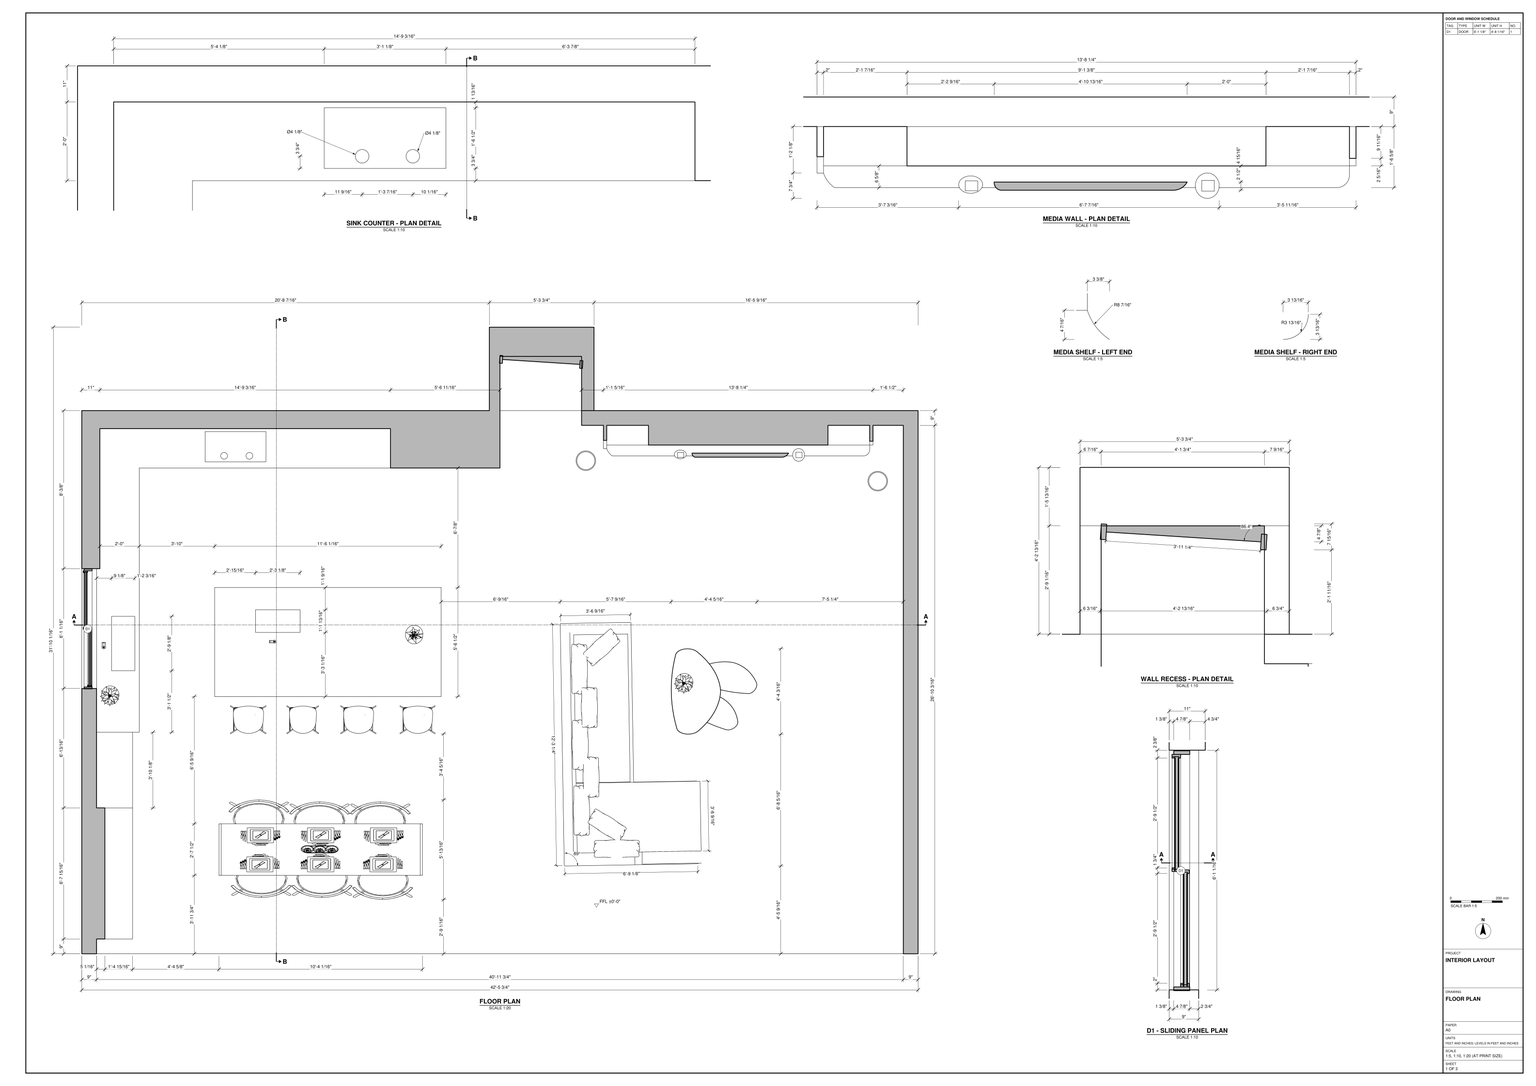
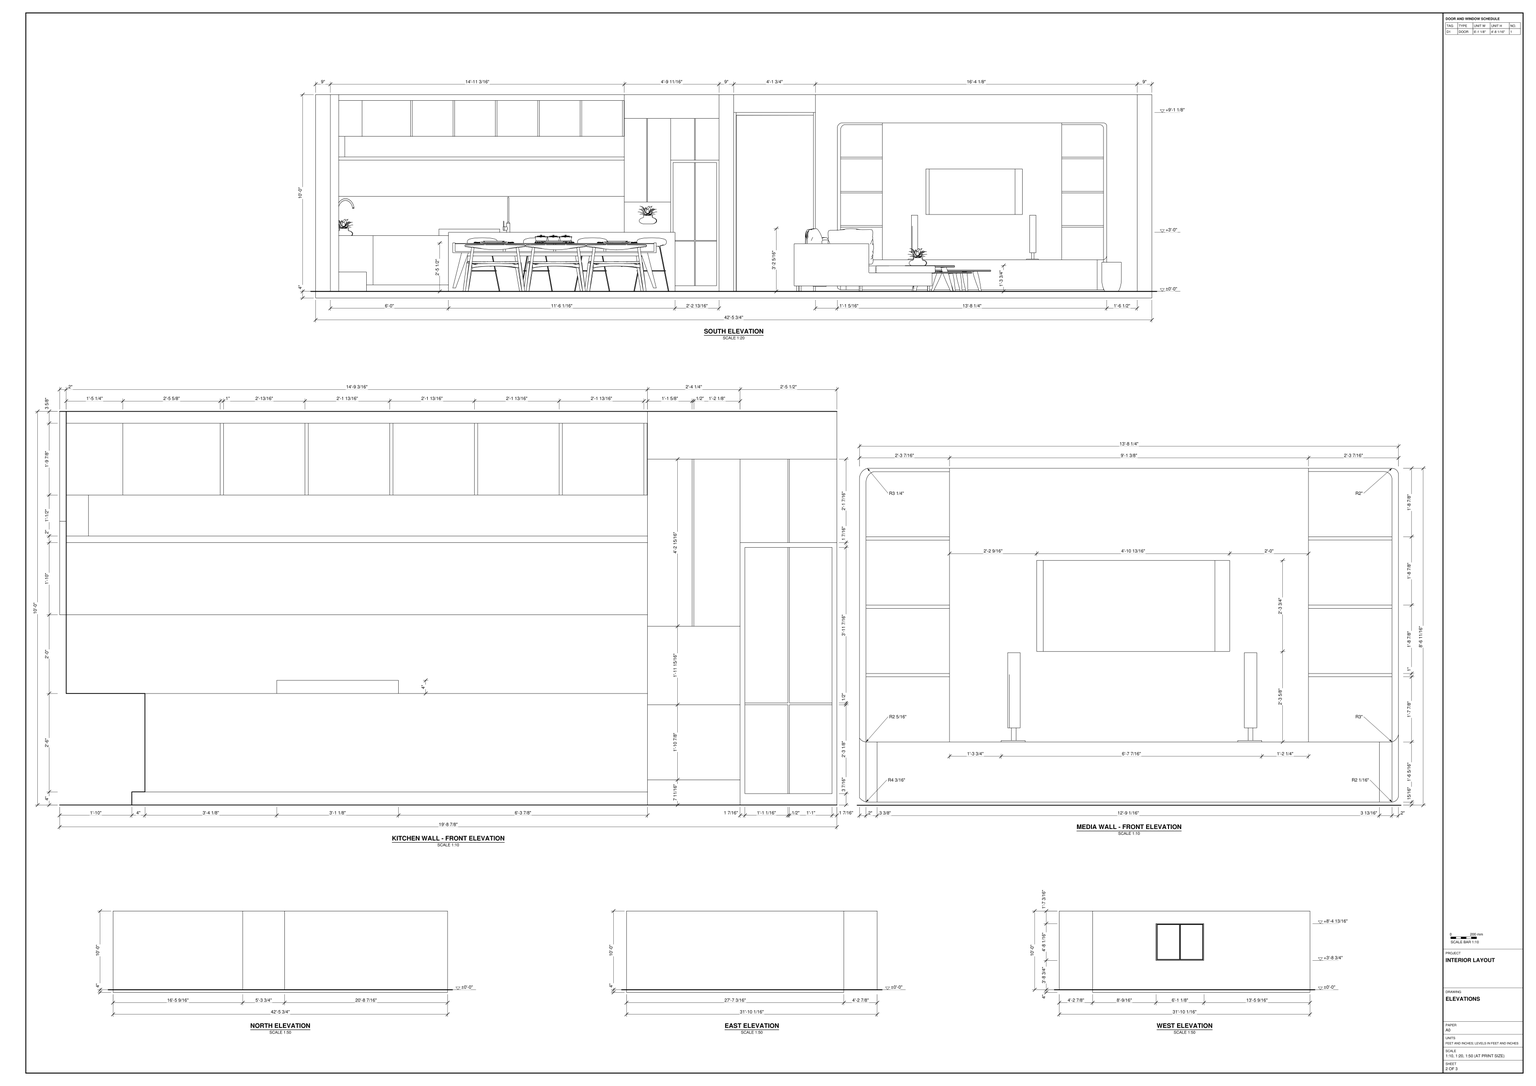
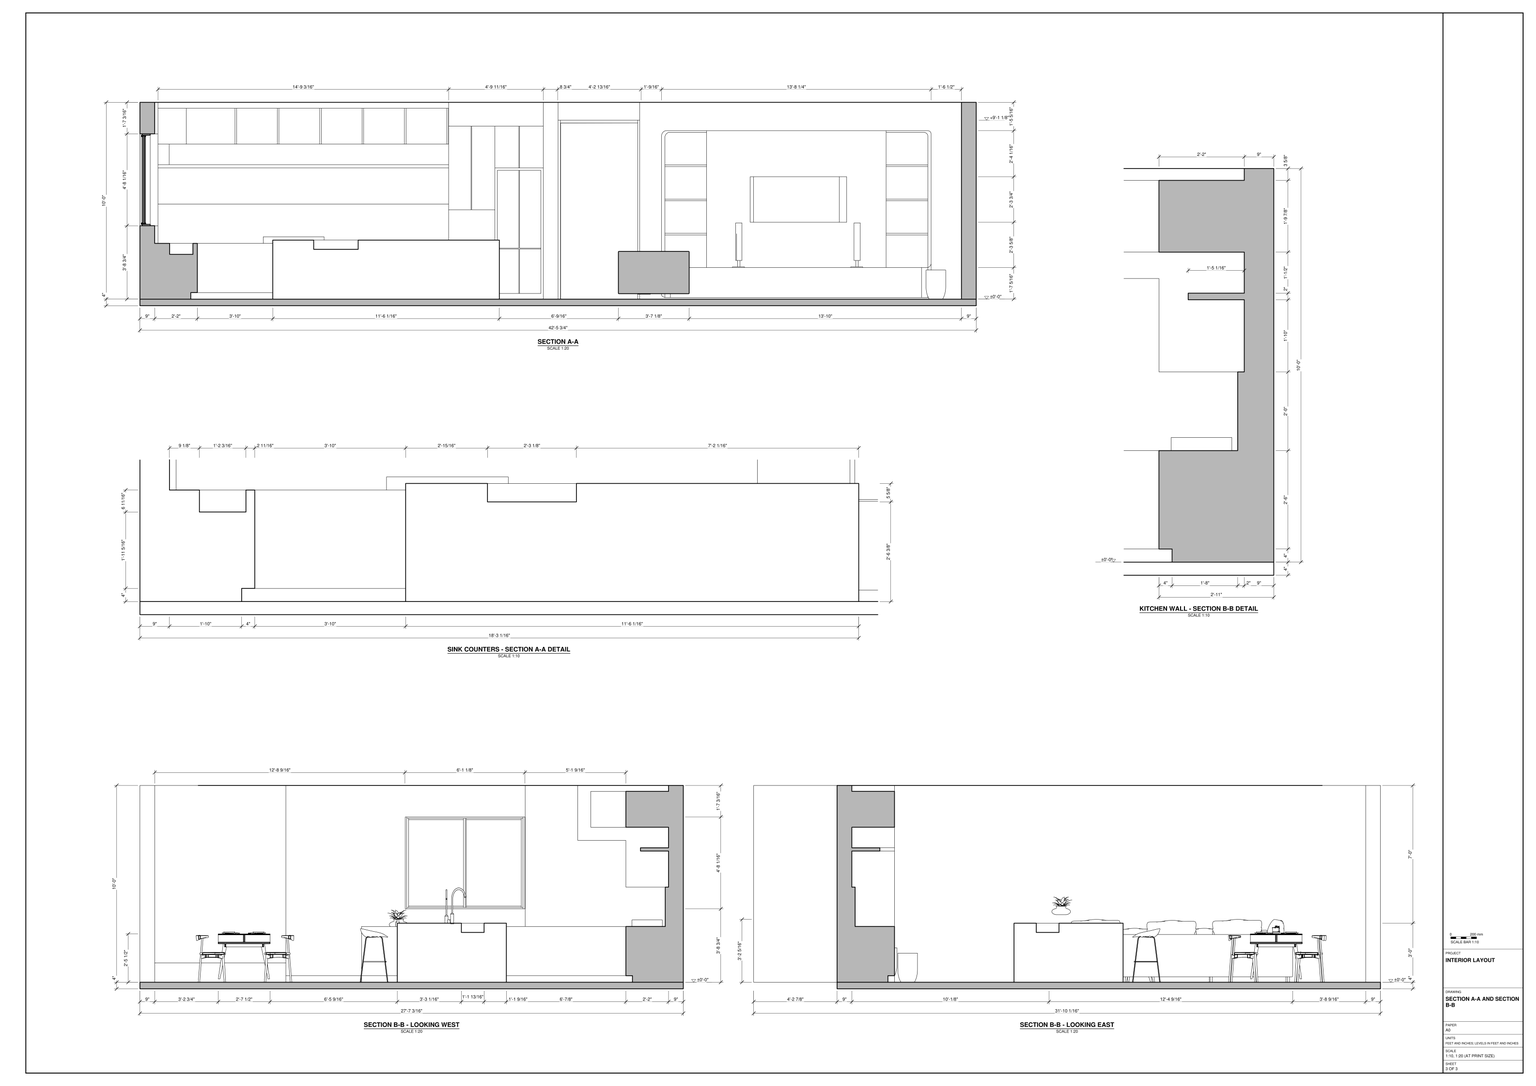
Build the interior shown in task_files/diagram_01.pdf as a single SketchUp model. Work in feet and inches. The overall extents are 42'-5 3/4" east to west, 31'-10 1/16" north to south and 10'-4" vertically. Set the finished floor at ±0'-0". Use the plan for the floor slab, wall returns and openings, and the sections for slab depth, wall heights and changes in wall thickness. Reproduce the projecting recess in the north wall and the framed sliding panels above the west counter.

Fit the kitchen into the northwest corner. Model the sink counter, the counter return, the upper cabinets, the shelf and the tall storage at the end of the cabinet run. Place the island parallel to the north counter, with the stools along its dining side. Set the dining table and chairs south of the island. In the living area, model the media wall with its low base, central display area and flanking shelves. Position the sectional sofa and low tables according to their footprints on the plan. Decor and loose items may be any suitable library components.

Keep the shell elements and each furniture or joinery piece in separate groups or components, and use components for repeated parts. Save the finished model as output_files/open_plan_kitchen_dining_and_living_interior.skp.

# SketchUp Ruby script. Lengths in inches.
U = 1.inch
M = Sketchup.active_model
def pt(a) = Geom::Point3d.new(a.map { |v| v * U })
def face(e, loops, mat)
  f = e.add_face(loops[0].map { |a| pt(a) })
  loops[1..].each { |l| e.add_face(l.map { |a| pt(a) }).erase! }
  f.material = f.back_material = mat if mat
  f
end
# faces: each face lists its corners as indices into pts; further lists are holes
def faces(e, pts, list, mat = nil) = list.each { |f| face(e, (f[0].is_a?(Array) ? f : [f]).map { |l| l.map { |i| pts[i] } }, mat) }
# xy, xz, yz: faces in a plane at the given z, y or x. An outline is a flat list of corners, or four numbers for a rectangle; further outlines are holes
def ring(l) = l.size == 4 ? [[l[0], l[1]], [l[2], l[1]], [l[2], l[3]], [l[0], l[3]]] : l.each_slice(2).to_a
def flat(e, list, mat, &to3) = list.each { |f| face(e, (f[0].is_a?(Array) ? f : [f]).map { |l| ring(l).map { |u, v| to3.(u, v) } }, mat) }
def xy(e, z, list, mat = nil) = flat(e, list, mat) { |x, y| [x, y, z] }
def xz(e, y, list, mat = nil) = flat(e, list, mat) { |x, z| [x, y, z] }
def yz(e, x, list, mat = nil) = flat(e, list, mat) { |y, z| [x, y, z] }
def lines(e, pts, list) = list.each { |a, b| e.add_line(pt(pts[a]), pt(pts[b])) }
# prism: a flat outline (further loops are holes) pulled along v
def prism(e, loops, v, mat = nil)
  f = face(e, loops, mat); d = Geom::Vector3d.new(v.map { |x| x * U })
  f.pushpull(f.normal.samedirection?(d) ? d.length : -d.length)
end
def box(e, o, s, mat = nil) = prism(e, [[o, [o[0] + s[0], o[1], o[2]], [o[0] + s[0], o[1] + s[1], o[2]], [o[0], o[1] + s[1], o[2]]]], [0, 0, s[2]], mat)
def at(x, y, z, deg = 0) = Geom::Transformation.translation(pt([x, y, z])) * Geom::Transformation.rotation(ORIGIN, Z_AXIS, deg.degrees)
def axes(o, x, y, z) = Geom::Transformation.new([*x, 0, *y, 0, *z, 0, *pt(o).to_a, 1])
def part(name) = M.definitions.add(name)
# library, detail: a bought-in or finely detailed component or shape, given as its bounding box
def library(name, o, s) = part(name).tap { |d| box(d.entities, o, s) }
def detail(e, o, s) = box(e.add_group.entities, o, s)
def put(e, d, t, mat = nil) = e.add_instance(d, t).tap { |i| i.material = mat if mat }
def group(e, t, mat = nil) = e.add_group.tap { |g| g.transformation = t; g.material = mat if mat }.entities
root = M.entities
M.materials.add("Generic\#1").color = [245, 240, 201]
M.materials.add("Glass_Mirror_01").color = [185, 185, 185]
M.materials.add("Glass_Tinted_Gray").color = [0, 0, 0]
M.materials["Glass_Tinted_Gray"].alpha = 0.125
M.materials.add("M07_Charcoal_Gleam").color = [58, 58, 58]
M.materials.add("Marble_07_1K").color = [36, 34, 36]
M.materials.add("Plywood_08_1K").color = [202, 166, 113]
M.materials.add("Polis06_194").color = [79, 50, 36]
M.materials.add("Wood_Floor_01_1K").color = [146, 111, 76]
M.materials.add("[0135_DarkGray]").color = [81, 81, 81]
M.materials.add("[Color_007]").color = [58, 58, 58]
M.materials.add("[Color_008]").color = [30, 30, 30]
M.materials.add("[Color_009]").color = [0, 0, 0]
M.materials.add("[Color_A01]").color = [255, 0, 0]
M.materials.add("[Mirror 02]").color = [229, 229, 229]
M.materials.add("[Terrazzo Light Blue]").color = [196, 214, 227]
c1 = library("tabouret",[40.37,22.21,0.38],[16.93,17.08,32.69])
c2 = library("Ikea_Ringskar.skp",[-1.97,-9.27,0],[4.06,9.27,15.35])
c3 = library("sofá dubai",[-3.2,-61.37,0],[197.52,171.62,48.7])
c4 = library("Dining table set",[0,0,0],[60.82,70.9,34.61])
c5 = part("Tv")
xy(c5.entities,0,[[2.03,0,1.74,0.06,1.46,0.15,1.19,0.27,0.95,0.43,0.72,0.62,0.52,0.84,0.35,1.08,0.21,1.34,0.1,1.61,0.03,1.9,0,2.19,0.01,2.48,59.41,2.48,59.17,2.1,58.9,1.74,58.59,1.41,58.25,1.1,57.89,0.83,57.5,0.6,57.09,0.4,56.67,0.24,56.23,0.12,55.78,0.04,55.33,0]],"[Color_009]")
xy(c5.entities,27.76,[[2.03,0,55.33,0,55.78,0.04,56.23,0.12,56.67,0.24,57.09,0.4,57.5,0.6,57.89,0.83,58.25,1.1,58.59,1.41,58.9,1.74,59.17,2.1,59.41,2.48,0.01,2.48,0,2.19,0.03,1.9,0.1,1.61,0.21,1.34,0.35,1.08,0.52,0.84,0.72,0.62,0.95,0.43,1.19,0.27,1.46,0.15,1.74,0.06]],"[Color_009]")
xz(c5.entities,0,[[2.03,0,54.875,27.76],[54.875,0,55.33,27.76]],"[Color_009]")
xz(c5.entities,2.48,[[0.69,0.6875,58.73,27.07]],"[Color_007]")
xz(c5.entities,2.48,[[[0.01,0,59.41,27.76],[0.69,0.6875,58.73,27.07],[5.81,0.12,5.86,0.12,5.91,0.13,5.99,0.19,6.03,0.29,6.03,0.34,6.01,0.39,5.99,0.43,5.95,0.47,5.91,0.5,5.86,0.51,5.81,0.51,5.76,0.5,5.71,0.47,5.65,0.39,5.64,0.34,5.64,0.29,5.65,0.24,5.68,0.19,5.71,0.16,5.76,0.13]]],"[Color_009]")
xz(c5.entities,2.48,[[5.81,0.12,5.76,0.13,5.71,0.16,5.68,0.19,5.65,0.24,5.64,0.29,5.64,0.34,5.65,0.39,5.71,0.47,5.76,0.5,5.81,0.51,5.86,0.51,5.91,0.5,5.95,0.47,5.99,0.43,6.01,0.39,6.03,0.34,6.03,0.29,5.99,0.19,5.91,0.13,5.86,0.12]],"[Color_A01]")
p = [[1.74,0.06,0],[2.03,0,0],[2.03,0,27.76],[1.74,0.06,27.76],[55.33,0,0],[55.78,0.04,0],
  [55.78,0.04,27.76],[55.33,0,27.76],[56.23,0.12,0],[56.23,0.12,27.76],[1.19,0.27,0],[1.46,0.15,0],
  [1.46,0.15,27.76],[1.19,0.27,27.76],[56.67,0.24,0],[56.67,0.24,27.76],[57.09,0.4,0],[57.09,0.4,27.76],
  [0.95,0.43,0],[0.95,0.43,27.76],[0.72,0.62,0],[0.72,0.62,27.76],[57.5,0.6,0],[57.5,0.6,27.76],
  [0.52,0.84,0],[0.52,0.84,27.76],[57.89,0.83,0],[57.89,0.83,27.76],[0.35,1.08,0],[0.35,1.08,27.76],
  [58.25,1.1,0],[58.25,1.1,27.76],[0.21,1.34,0],[0.21,1.34,27.76],[58.59,1.41,0],[58.59,1.41,27.76],
  [0.1,1.61,0],[0.1,1.61,27.76],[58.9,1.74,0],[58.9,1.74,27.76],[0.03,1.9,0],[0.03,1.9,27.76],
  [59.17,2.1,0],[59.17,2.1,27.76],[0,2.19,0],[0,2.19,27.76],[59.41,2.48,0],[59.41,2.48,27.76],
  [0.01,2.48,0],[0.01,2.48,27.76]]
faces(c5.entities,p,[[0,1,2,3],[4,5,6,7],[5,8,9,6],[10,11,12,13],[11,0,3,12],[8,14,15,9],[14,16,17,15],[18,10,13,19],
  [20,18,19,21],[16,22,23,17],[24,20,21,25],[22,26,27,23],[28,24,25,29],[26,30,31,27],[32,28,29,33],[30,34,35,31],
  [36,32,33,37],[34,38,39,35],[40,36,37,41],[38,42,43,39],[44,40,41,45],[42,46,47,43],[48,44,45,49]],"[Color_009]")
c6 = part("Televisão")
xy(c6.entities,0,[[76.54,0.53,75.59,0.66,74.69,1.05,73.93,1.66,73.34,2.47,72.97,3.4,72.84,4.41,72.97,5.42,73.34,6.35,73.93,7.16,74.69,7.77,75.59,8.16,76.54,8.29,77.5,8.16,78.39,7.77,79.16,7.16,79.75,6.35,80.12,5.42,80.24,4.41,80.12,3.4,79.75,2.47,79.16,1.66,78.39,1.05,77.5,0.66],[3.7,2.07,2.74,2.16,1.85,2.43,1.08,2.85,0.5,3.4,0.125,4.05,0,4.74,0.125,5.43,0.5,6.07,1.08,6.62,1.85,7.04,2.74,7.3125,3.7,7.4,4.66,7.3125,5.55,7.04,6.32,6.62,6.91,6.07,7.28,5.43,7.4,4.74,7.28,4.05,6.91,3.4,6.32,2.85,5.55,2.43,4.66,2.16]],"[Color_009]")
xy(c6.entities,0.43,[[[76.54,0.53,77.5,0.66,78.39,1.05,79.16,1.66,79.75,2.47,80.12,3.4,80.24,4.41,80.12,5.42,79.75,6.35,79.16,7.16,78.39,7.77,77.5,8.16,76.54,8.29,75.59,8.16,74.69,7.77,73.93,7.16,73.34,6.35,72.97,5.42,72.84,4.41,72.97,3.4,73.34,2.47,73.93,1.66,74.69,1.05,75.59,0.66],[76.03,3.29,77.48,5.48]],[[3.7,2.07,4.66,2.16,5.55,2.43,6.32,2.85,6.91,3.4,7.28,4.05,7.4,4.74,7.28,5.43,6.91,6.07,6.32,6.62,5.55,7.04,4.66,7.3125,3.7,7.4,2.74,7.3125,1.85,7.04,1.08,6.62,0.5,6.07,0.125,5.43,0,4.74,0.125,4.05,0.5,3.4,1.08,2.85,1.85,2.43,2.74,2.16],[3.18,3.97,4.64,5.47]]],"[Color_008]")
xy(c6.entities,4.29,[[[74.87,2.73,78.72,6.04],[76.03,3.29,77.48,5.48]],[[2.02,2.86,5.88,5.85],[3.18,3.97,4.64,5.47]]],"[Color_009]")
xy(c6.entities,27.2,[[74.87,2.73,78.72,6.04],[2.02,2.86,5.88,5.85]],"[Color_009]")
xz(c6.entities,2.73,[[74.87,4.29,78.72,27.2]],"[Color_009]")
xz(c6.entities,2.86,[[2.02,4.29,5.88,27.2]],"[Color_009]")
xz(c6.entities,3.29,[[76.03,0.43,77.48,4.29]],"[Color_009]")
xz(c6.entities,3.97,[[3.18,0.43,4.64,4.29]],"[Color_009]")
xz(c6.entities,5.47,[[3.18,0.43,4.64,4.29]],"[Color_009]")
xz(c6.entities,5.48,[[76.03,0.43,77.48,4.29]],"[Color_009]")
xz(c6.entities,5.85,[[2.17,4.44,5.73,27.06]],"[Color_007]")
xz(c6.entities,5.85,[[[2.02,4.29,5.88,27.2],[2.17,4.44,5.73,27.06]]],"[Color_009]")
xz(c6.entities,6.04,[[75.01,4.44,78.58,27.06]],"[Color_007]")
xz(c6.entities,6.04,[[[74.87,4.29,78.72,27.2],[75.01,4.44,78.58,27.06]]],"[Color_009]")
yz(c6.entities,2.02,[[2.86,4.29,5.85,27.2]],"[Color_009]")
yz(c6.entities,3.18,[[3.97,0.43,5.47,4.29]],"[Color_009]")
yz(c6.entities,4.64,[[3.97,0.43,5.47,4.29]],"[Color_009]")
yz(c6.entities,5.88,[[2.86,4.29,5.85,27.2]],"[Color_009]")
yz(c6.entities,74.87,[[2.73,4.29,6.04,27.2]],"[Color_009]")
yz(c6.entities,76.03,[[3.29,0.43,5.48,4.29]],"[Color_009]")
yz(c6.entities,77.48,[[3.29,0.43,5.48,4.29]],"[Color_009]")
yz(c6.entities,78.72,[[2.73,4.29,6.04,27.2]],"[Color_009]")
p = [[75.59,0.66,0],[76.54,0.53,0],[76.54,0.53,0.43],[75.59,0.66,0.43],[77.5,0.66,0],[77.5,0.66,0.43],
  [74.69,1.05,0],[74.69,1.05,0.43],[78.39,1.05,0],[78.39,1.05,0.43],[73.93,1.66,0],[73.93,1.66,0.43],
  [79.16,1.66,0],[79.16,1.66,0.43],[73.34,2.47,0],[73.34,2.47,0.43],[79.75,2.47,0],[79.75,2.47,0.43],
  [2.74,2.16,0],[3.7,2.07,0],[3.7,2.07,0.43],[2.74,2.16,0.43],[4.66,2.16,0],[4.66,2.16,0.43],
  [1.85,2.43,0],[1.85,2.43,0.43],[5.55,2.43,0],[5.55,2.43,0.43],[1.08,2.85,0],[1.08,2.85,0.43],
  [6.32,2.85,0],[6.32,2.85,0.43],[72.97,3.4,0],[72.97,3.4,0.43],[80.12,3.4,0],[80.12,3.4,0.43],
  [0.5,3.4,0],[0.5,3.4,0.43],[6.91,3.4,0],[6.91,3.4,0.43],[0.125,4.05,0],[0.125,4.05,0.43],
  [7.28,4.05,0],[7.28,4.05,0.43],[72.84,4.41,0],[72.84,4.41,0.43],[80.24,4.41,0],[80.24,4.41,0.43],
  [0,4.74,0],[0,4.74,0.43],[7.4,4.74,0],[7.4,4.74,0.43],[72.97,5.42,0],[72.97,5.42,0.43],
  [80.12,5.42,0],[80.12,5.42,0.43],[0.125,5.43,0],[0.125,5.43,0.43],[7.28,5.43,0],[7.28,5.43,0.43],
  [0.5,6.07,0],[0.5,6.07,0.43],[6.91,6.07,0],[6.91,6.07,0.43],[73.34,6.35,0],[73.34,6.35,0.43],
  [79.75,6.35,0],[79.75,6.35,0.43],[1.08,6.62,0],[1.08,6.62,0.43],[6.32,6.62,0],[6.32,6.62,0.43],
  [73.93,7.16,0],[73.93,7.16,0.43],[79.16,7.16,0],[79.16,7.16,0.43],[1.85,7.04,0],[1.85,7.04,0.43],
  [5.55,7.04,0],[5.55,7.04,0.43],[2.74,7.3125,0],[2.74,7.3125,0.43],[4.66,7.3125,0],[4.66,7.3125,0.43],
  [74.69,7.77,0],[74.69,7.77,0.43],[78.39,7.77,0],[78.39,7.77,0.43],[3.7,7.4,0],[3.7,7.4,0.43],
  [75.59,8.16,0],[75.59,8.16,0.43],[77.5,8.16,0],[77.5,8.16,0.43],[76.54,8.29,0],[76.54,8.29,0.43],
  [75.4,3.53,4.29],[75.4,3.53,20.55],[77.48,5.48,4.29],[77.48,5.48,20.55],[75.4,5.61,4.29],[75.4,5.61,20.55],
  [2.55,2.63,4.29],[2.55,2.63,20.55],[4.64,5.47,4.29],[4.64,5.47,20.55],[2.55,4.72,4.29],[2.55,4.72,20.55]]
faces(c6.entities,p,[[0,1,2,3],[1,4,5,2],[6,0,3,7],[4,8,9,5],[10,6,7,11],[8,12,13,9],[14,10,11,15],[12,16,17,13],
  [18,19,20,21],[19,22,23,20],[24,18,21,25],[22,26,27,23],[28,24,25,29],[26,30,31,27],[32,14,15,33],[16,34,35,17],
  [36,28,29,37],[30,38,39,31],[40,36,37,41],[38,42,43,39],[44,32,33,45],[34,46,47,35],[48,40,41,49],[42,50,51,43],
  [52,44,45,53],[46,54,55,47],[56,48,49,57],[50,58,59,51],[60,56,57,61],[58,62,63,59],[64,52,53,65],[54,66,67,55],
  [68,60,61,69],[62,70,71,63],[72,64,65,73],[66,74,75,67],[76,68,69,77],[70,78,79,71],[80,76,77,81],[78,82,83,79],
  [84,72,73,85],[74,86,87,75],[88,80,81,89],[82,88,89,83],[90,84,85,91],[86,92,93,87],[94,90,91,95],[92,94,95,93]],"[Color_009]")
lines(c6.entities,p,[[96,97],[98,99],[100,101],[102,103],[104,105],[106,107]])
put(c6.entities,c5,at(10.94,3.03,27.6))
c7 = part("PENTEK_RP Fineline 50S_Sliding_DoorCase_E1")
box(c7.entities,[0,0,0],[1.51,3.66,99.27],"[0135_DarkGray]")
c8 = part("PENTEK_RP Fineline 50S_SlidingDooe_Case_E2")
box(c8.entities,[0,0,0],[96.25,3.66,1.51],"[0135_DarkGray]")
c9 = part("pentek_RP Fineline 50S_SlidingDoor_Case")
put(c9.entities,c7,at(97.76,0,0))
put(c9.entities,c8,at(1.51,0,0))
put(c9.entities,c7,at(0,0,0))
put(c9.entities,c8,at(1.51,0,97.76))
c10 = part("PENTEK_RP Fineline 50S_SlidingDoor_GlazingBead_2")
box(c10.entities,[0,0,0],[0.56,0.59,94.39],"[0135_DarkGray]")
c11 = part("PENTEK_RP Fineline 50S_SlidingDoor_Glass")
box(c11.entities,[0,0,0],[46.58,0.16,94.39],"Glass_Tinted_Gray")
c12 = part("PENTEK_RP Fineline 50S_SlidingDoor_GlazingBead")
box(c12.entities,[0,0,0],[45.47,0.59,0.56],"[0135_DarkGray]")
c13 = part("PENTEK_RP Fineline 50S_SlidingDoor_Leaf_E1")
xy(c13.entities,0,[[0,0,0.93,1.97],[0.93,1.57,1.49,1.97]],"[0135_DarkGray]")
xy(c13.entities,96.25,[[0,0,0.93,0,0.93,1.57,1.49,1.57,1.49,1.97,0,1.97]],"[0135_DarkGray]")
xz(c13.entities,0,[[0,0,0.93,96.25]],"[0135_DarkGray]")
xz(c13.entities,1.57,[[0.93,0,1.49,95.32],[0.93,95.32,1.49,96.25]],"[0135_DarkGray]")
xz(c13.entities,1.97,[[0,0,1.49,96.25]],"[0135_DarkGray]")
yz(c13.entities,0,[[0,0,1.97,96.25]],"[0135_DarkGray]")
yz(c13.entities,0.93,[[0,0,1.57,0.93],[0,0.93,1.57,95.32],[0,95.32,1.57,96.25]],"[0135_DarkGray]")
yz(c13.entities,1.49,[[1.57,0,1.97,95.32],[1.57,95.32,1.97,96.25]],"[0135_DarkGray]")
c14 = part("PENTEK_RP Fineline 50S_SlidingDoor_Leaf_E2")
xy(c14.entities,0,[[0,0,0,1.57,0.56,1.57,0.56,1.97,46.02,1.97,46.02,1.57,46.58,1.57,46.58,0]],"[0135_DarkGray]")
xy(c14.entities,0.93,[[0,0,46.58,1.57]],"[0135_DarkGray]")
xy(c14.entities,1.49,[[0.56,1.57,46.02,1.97]],"[0135_DarkGray]")
xz(c14.entities,0,[[0,0,46.58,0.93]],"[0135_DarkGray]")
xz(c14.entities,1.57,[[0,0,0.56,0.93],[46.02,0,46.58,0.93],[0.56,0.93,46.02,1.49]],"[0135_DarkGray]")
xz(c14.entities,1.97,[[0.56,0,46.02,1.49]],"[0135_DarkGray]")
yz(c14.entities,0,[[0,0,1.57,0.93]],"[0135_DarkGray]")
yz(c14.entities,0.56,[[1.57,0,1.97,0.93],[1.57,0.93,1.97,1.49]],"[0135_DarkGray]")
yz(c14.entities,46.02,[[1.57,0,1.97,0.93],[1.57,0.93,1.97,1.49]],"[0135_DarkGray]")
yz(c14.entities,46.58,[[0,0,1.57,0.93]],"[0135_DarkGray]")
c15 = part("PENTEK_RP Fineline S_SlidingDoor_Leaf1")
put(c15.entities,c10,at(0.93,0,0.93))
put(c15.entities,c10,at(46.96,0,0.93))
put(c15.entities,c11,at(1.49,1.42,0.93))
put(c15.entities,c12,at(1.49,0,0.93))
put(c15.entities,c11,at(1.49,0.59,0.93),"[Terrazzo Light Blue]")
put(c15.entities,c13,at(0,0,0))
put(c15.entities,c13,axes([48.44,0,0],[-1,0,0],[0,1,0],[0,0,1]))
put(c15.entities,c14,axes([0.93,0,96.25],[1,0,0],[0,1,0],[0,0,-1]))
put(c15.entities,c14,at(0.93,0,0))
put(c15.entities,c12,at(1.49,0,94.77))
c16 = part("PENTEK_RP Fineline 50S_SlidingDoor_Leaf2")
put(c16.entities,c11,at(1.49,1.42,0.93))
put(c16.entities,c12,at(1.49,0,94.77))
put(c16.entities,c10,at(46.96,0,0.93))
put(c16.entities,c11,at(1.49,0.59,0.93),"[Mirror 02]")
put(c16.entities,c10,at(0.93,0,0.93))
put(c16.entities,c13,at(0,0,0))
put(c16.entities,c13,axes([48.44,0,0],[-1,0,0],[0,1,0],[0,0,1]))
put(c16.entities,c12,at(1.49,0,0.93))
put(c16.entities,c14,axes([0.93,0,96.25],[1,0,0],[0,1,0],[0,0,-1]))
put(c16.entities,c14,at(0.93,0,0))
c17 = part("PENTEK - Slimmest Steel Sliding Door / Window\#1")
put(c17.entities,c9,at(0,-1.88,-0.09))
put(c17.entities,c15,at(1.51,-2.27,1.42))
put(c17.entities,c16,at(49.32,-0.3,1.42))
c18 = part("Interior door")
xy(c18.entities,0,[[0,0,4.72,1.18],[0,34.25,4.72,35.43]],"Polis06_194")
xy(c18.entities,85.26,[[0,1.18,4.72,34.25]],"Polis06_194")
xy(c18.entities,86.61,[[0,0,4.72,35.43]],"Polis06_194")
xz(c18.entities,0,[[0,0,4.72,86.61]],"Polis06_194")
xz(c18.entities,1.18,[[0,0,2.36,85.26],[2.36,0,4.72,85.26]],"Polis06_194")
xz(c18.entities,34.25,[[0,0,4.72,85.26]],"Polis06_194")
xz(c18.entities,35.43,[[0,0,4.72,86.61]],"Polis06_194")
yz(c18.entities,0,[[0,0,1.18,86.61],[34.25,0,35.43,86.61],[1.18,85.26,34.25,86.61]],"Polis06_194")
yz(c18.entities,2.36,[[1.18,0,34.25,0,34.25,85.21,1.18,85.26]],"Polis06_194")
yz(c18.entities,4.72,[[0,0,1.18,86.61],[34.25,0,35.43,86.61],[1.18,85.26,34.25,86.61]],"Polis06_194")
c19 = library("Group_432",[-8.27,-1.37,0],[9.69,9.67,11.03])
c20 = library("Flower_pot+09",[-33.27,-15.12,-0.3125],[11.99,12,18.05])
xy(root,4,[[0,0,9,0,9,9,14.0625,9,14.0625,88.95,9,88.95,9,135.09,31,135.09,31,300.2,188.16,300.2,188.16,296.2,254.87,296.2,254.87,331.2,0,331.2],[500.74,0,509.74,0,509.74,331.2,304.63,331.2,304.63,322.2,500.74,322.2],[80.98,156.87,219.0625,223.35],[248.43,331.2,254.87,364.25],[304.63,331.2,312.19,364.25],
  [248.43,364.25,312.19,382.05]])
xy(root,4.96,[[323.35,303.58,322.96,303.85,322.58,304.15,322.23,304.46,321.89,304.79,321.57,305.15,321.28,305.51,321,305.9,320.75,306.3,320.51,306.71,320.31,307.14,320.12,307.57,319.96,308.02,319.96,322.2,480.24,322.2,480.24,307.42,480.21,306.92,480.11,306.43,479.95,305.95,479.73,305.5,479.45,305.08,479.12,304.71,478.74,304.375,478.32,304.1,477.87,303.875,477.39,303.71,476.9,303.61,476.4,303.58]],"Wood_Floor_01_1K")
xy(root,8,[[31,135.09,35,300.2],[35,296.2,188.16,300.2]])
xy(root,8,[[9,88.95,31,135.09]],"Generic\#1")
xy(root,15.8,[[14.0625,9,31,88.95]],"Generic\#1")
xy(root,23.28,[[323.35,303.58,476.4,303.58,476.9,303.61,477.39,303.71,477.87,303.875,478.32,304.1,478.74,304.375,479.12,304.71,479.45,305.08,479.73,305.5,479.95,305.95,480.11,306.43,480.21,306.92,480.24,307.42,480.24,322.2,454.8,322.2,454.8,310.2,345.4,310.2,345.4,322.2,319.96,322.2,319.96,308.02,320.12,307.57,320.31,307.14,320.51,306.71,320.75,306.3,321,305.9,321.28,305.51,321.57,305.15,321.89,304.79,322.23,304.46,322.58,304.15,322.96,303.85]],"Generic\#1")
xy(root,31.29,[[18.125,172.6,32.31,205.75]],"Marble_07_1K")
xy(root,34.38,[[105.92,195.9375,133.02,209.78]],"Marble_07_1K")
xy(root,38,[[[9,135.09,35,135.09,35,296.2,188.16,296.2,188.16,320.2,11,320.2,11,234.83,9,234.83],[75.15,299.93,112.26,318.42],[18.125,172.6,32.31,205.75]]],"Generic\#1")
xy(root,40,[[[80.98,156.87,219.0625,223.35],[105.92,195.9375,133.02,209.78]]],"Generic\#1")
xy(root,42,[[86.73,301.57,87.26,301.64,87.76,301.84,88.19,302.17,88.52,302.6,88.73,303.1,88.8,303.64,88.73,304.18,88.52,304.68,88.19,305.11,87.76,305.4375,87.26,305.64,86.73,305.71,86.19,305.64,85.69,305.4375,85.26,305.11,84.93,304.68,84.72,304.18,84.65,303.64,84.72,303.1,84.93,302.6,85.26,302.17,85.69,301.84,86.19,301.64],[102.17,301.57,102.71,301.64,103.21,301.84,103.64,302.17,103.97,302.6,104.17,303.1,104.25,303.64,104.17,304.18,103.97,304.68,103.64,305.11,103.21,305.4375,102.71,305.64,102.17,305.71,101.63,305.64,101.13,305.4375,100.7,305.11,100.375,304.68,100.17,304.18,100.1,303.64,100.17,303.1,100.375,302.6,100.7,302.17,101.13,301.84,101.63,301.64]])
xy(root,42,[[[75.15,299.93,112.26,318.42],[102.17,301.57,101.63,301.64,101.13,301.84,100.7,302.17,100.375,302.6,100.17,303.1,100.1,303.64,100.17,304.18,100.375,304.68,100.7,305.11,101.13,305.4375,101.63,305.64,102.17,305.71,102.71,305.64,103.21,305.4375,103.64,305.11,103.97,304.68,104.17,304.18,104.25,303.64,104.17,303.1,103.97,302.6,103.64,302.17,103.21,301.84,102.71,301.64],[86.73,301.57,86.19,301.64,85.69,301.84,85.26,302.17,84.93,302.6,84.72,303.1,84.65,303.64,84.72,304.18,84.93,304.68,85.26,305.11,85.69,305.4375,86.19,305.64,86.73,305.71,87.26,305.64,87.76,305.4375,88.19,305.11,88.52,304.68,88.73,304.18,88.8,303.64,88.73,303.1,88.52,302.6,88.19,302.17,87.76,301.84,87.26,301.64]]],"M07_Charcoal_Gleam")
xy(root,43.13,[[319.96,310.2,345.4,322.2]],"Wood_Floor_01_1K")
xy(root,43.14,[[454.8,310.2,480.24,322.2]],"Wood_Floor_01_1K")
xy(root,44.13,[[319.96,310.2,345.4,322.2]],"Wood_Floor_01_1K")
xy(root,44.14,[[454.8,310.2,480.24,322.2]],"Wood_Floor_01_1K")
xy(root,48.75,[[0,161.75,9,234.83]])
xy(root,62,[[9,296.2,11,320.2]])
xy(root,62,[[9,320.2,188.16,322.2]],"Generic\#1")
xy(root,63.98,[[319.96,310.2,345.4,322.2]],"Wood_Floor_01_1K")
xy(root,64,[[454.8,310.2,480.24,322.2]],"Wood_Floor_01_1K")
xy(root,64.98,[[319.96,310.2,345.4,322.2]],"Wood_Floor_01_1K")
xy(root,65,[[454.8,310.2,480.24,322.2]],"Wood_Floor_01_1K")
xy(root,84,[[9,305.11,188.16,322.2]])
xy(root,84.83,[[319.96,310.2,345.4,322.2]],"Wood_Floor_01_1K")
xy(root,84.86,[[454.8,310.2,480.24,322.2]],"Wood_Floor_01_1K")
xy(root,85.83,[[319.96,310.2,345.4,322.2]],"Wood_Floor_01_1K")
xy(root,85.86,[[454.8,310.2,480.24,322.2]],"Wood_Floor_01_1K")
xy(root,86,[[9,305.11,188.16,322.2]],"Plywood_08_1K")
xy(root,90.48,[[9,266.89,11,280.8125],[9,280.8125,11,296.2]])
xy(root,98.51,[[9,274.79,11,280.8125],[11,274.79,28.28,296.2],[9,280.8125,11,296.2],[9,296.2,188.16,322.2]])
xy(root,104.8,[[0,161.75,9,234.83]])
xy(root,105.68,[[322.21,313.01,345.4,322.2]],"Wood_Floor_01_1K")
xy(root,105.72,[[454.8,312.5,477.82,322.2]],"Wood_Floor_01_1K")
xy(root,106.72,[[345.4,310.2,454.8,322.2],[454.8,312.5,480.24,322.2],[320.36,313.01,345.4,322.2]],"Wood_Floor_01_1K")
xy(root,120.39,[[9,274.79,28.28,274.79,28.28,296.2,188.16,296.2,188.16,322.2,9,322.2]],"Generic\#1")
xy(root,124,[[14.0625,35.51,500.74,35.51,500.74,322.2,304.63,322.2,304.63,331.2,254.87,331.2,254.87,296.2,188.16,296.2,188.16,322.2,9,322.2,9,266.89,11,266.89,11,234.83,9,234.83,9,88.95,14.0625,88.95],[254.87,331.2,304.63,364.25]])
xy(root,124,[[0,0,9,0,9,9,14.0625,9,14.0625,35.51,0,35.51],[500.74,0,509.74,35.51],[0,35.51,14.0625,35.51,14.0625,88.95,9,88.95,9,234.83,11,234.83,11,266.89,9,266.89,9,322.2,188.16,322.2,188.16,296.2,245.87,296.2,245.87,322.2,254.87,322.2,254.87,331.2,0,331.2],[500.74,35.51,509.74,35.51,509.74,331.2,304.63,331.2,304.63,322.2,500.74,322.2],[245.87,296.2,254.87,322.2],
  [248.43,331.2,254.87,331.2,254.87,364.25,304.63,364.25,304.63,331.2,312.19,331.2,312.19,382.05,248.43,382.05]],"Generic\#1")
xz(root,0,[[0,4,9,124],[500.74,4,509.74,124]],"Generic\#1")
xz(root,9,[[9,4,14.0625,124],[14.0625,4,31,15.8]],"Generic\#1")
xz(root,88.95,[[9,4,14.0625,8],[9,8,14.0625,124],[14.0625,8,31,15.8]])
xz(root,135.09,[[9,4,31,8]])
xz(root,135.09,[[9,8,35,38]],"Generic\#1")
xz(root,156.87,[[80.98,4,219.0625,40]],"Generic\#1")
xz(root,161.75,[[0,48.75,9,104.8]])
xz(root,172.6,[[18.125,31.29,32.31,38]])
xz(root,195.9375,[[105.92,34.38,133.02,40]],"Generic\#1")
xz(root,205.75,[[18.125,31.29,32.31,38]],"Marble_07_1K")
xz(root,209.78,[[105.92,34.38,133.02,40]],"Generic\#1")
xz(root,223.35,[[80.98,4,219.0625,40]],"Generic\#1")
xz(root,234.83,[[9,38,11,48.75],[0,48.75,4.5,104.8],[4.5,48.75,11,104.8],[9,104.8,11,124]])
xz(root,266.89,[[9,90.48,11,124]])
xz(root,274.79,[[9,98.51,28.28,120.39]],"Generic\#1")
xz(root,296.2,[[201.77,58.51,202.27,109.45],[9,62,11,90.48],[230.94,84,231.44,109.45],[57.93,98.51,58.93,120.39],[83.75,98.51,84.75,120.39],
  [109.58,98.51,110.58,120.39],[135.4,98.51,136.4,120.39],[161.22,98.51,162.22,120.39],[187.04,98.51,188.04,120.39],[188.04,98.51,188.16,120.39]])
xz(root,296.2,[[188.16,4,216.38,11.68],[245.87,4,254.87,124],[35,8,188.16,38],[188.16,58.51,201.77,109.45],[202.27,58.51,216.38,109.45],
  [216.38,84,230.94,109.45],[231.44,84,245.87,109.45],[28.28,98.51,57.93,120.39],[58.93,98.51,83.75,120.39],[84.75,98.51,109.58,120.39],
  [110.58,98.51,135.4,120.39],[136.4,98.51,161.22,120.39],[162.22,98.51,187.04,120.39],[188.16,109.45,245.87,124]],"Generic\#1")
xz(root,296.2,[[217.85,7.46,230.94,34.58],[231.44,7.46,244.41,34.58],[188.16,11.68,216.38,34.58],[188.16,34.58,216.38,58.51],[217.85,35.09,230.94,82.54],
  [231.44,35.09,244.41,82.54]],"Glass_Mirror_01")
xz(root,296.2,[[[216.38,4,245.87,84],[217.85,7.46,244.41,82.54]],[230.94,7.46,231.44,7.46,231.44,34.58,244.41,34.58,244.41,35.09,231.44,35.09,231.44,82.54,230.94,82.54,230.94,35.09,217.85,35.09,217.85,34.58,230.94,34.58]],"Marble_07_1K")
xz(root,299.93,[[75.15,38,112.26,42]],"M07_Charcoal_Gleam")
xz(root,300.2,[[31,4,188.16,8]],"Generic\#1")
xz(root,303.58,[[323.35,4.96,476.4,23.28]],"Generic\#1")
xz(root,305.11,[[9,84,188.16,86]],"Plywood_08_1K")
xz(root,308.02,[[319.96,4.96,319.96,23.28,319.76,23.3,319.56,23.33,319.36,23.38,319.16,23.45,318.98,23.53,318.8,23.63,318.63,23.75,318.47,23.88,318.32,24.02,318.1875,24.18,318.07,24.34,317.96,24.52,317.96,6.28,318.24,5.98,318.54,5.72,318.7,5.59,319.04,5.37,319.21,5.27,319.4,5.18,319.58,5.1]],"Generic\#1")
xz(root,310.2,[[345.4,23.28,454.8,106.72]],"Generic\#1")
xz(root,310.2,[[480.24,4.96,480.5,4.98,480.76,5.04,481.01,5.13,481.24,5.25,481.46,5.4,481.66,5.57,481.83,5.77,481.97,5.99,482.09,6.23,482.17,6.48,482.22,6.74,482.24,7,482.24,25.61,482.18,25.35,482.1,25.1,482,24.85,481.87,24.61,481.73,24.38,481.5625,24.17,481.38,23.98,481.18,23.8,480.96,23.64,480.73,23.5,480.49,23.38,480.24,23.28],[319.96,43.13,345.4,44.13],[454.8,43.14,480.24,44.14],[319.96,63.98,345.4,64.98],[454.8,64,480.24,65],
  [319.96,84.83,345.4,85.83],[454.8,84.86,480.24,85.86]],"Wood_Floor_01_1K")
xz(root,312.5,[[480.24,23.28,480.49,23.38,480.73,23.5,480.96,23.64,481.18,23.8,481.38,23.98,481.5625,24.17,481.73,24.38,481.87,24.61,482,24.85,482.1,25.1,482.18,25.35,482.24,25.61,482.24,104.72,482.22,104.98,482.17,105.23,482.09,105.48,481.97,105.72,481.83,105.93,481.65,106.13,481.46,106.3,481.24,106.45,481,106.56,480.76,106.65,480.5,106.7,480.24,106.72,454.8,106.72,454.8,105.72,477.82,105.72,478.1,105.7,478.39,105.65,478.66,105.57,478.93,105.45,479.18,105.3,479.41,105.13,479.62,104.93,479.8,104.71,479.96,104.46,480.08,104.21,480.18,103.93,480.24,103.65]],"Wood_Floor_01_1K")
xz(root,313.01,[[319.96,23.28,319.96,102.5,319.98,102.84,320.03,103.18,320.12,103.52,320.24,103.84,320.4,104.15,320.58,104.45,320.79,104.72,321.03,104.97,321.3,105.19,321.58,105.39,321.89,105.55,322.21,105.68,345.4,105.68,345.4,106.72,320.36,106.72,320.02,106.6,319.7,106.46,319.4,106.27,319.12,106.06,318.86,105.82,318.63,105.55,318.43,105.25,318.26,104.94,318.13,104.61,318.04,104.27,317.98,103.92,317.96,103.57,317.96,24.52,318.07,24.34,318.1875,24.18,318.32,24.02,318.47,23.88,318.63,23.75,318.8,23.63,318.98,23.53,319.16,23.45,319.36,23.38,319.56,23.33,319.76,23.3]],"Generic\#1")
xz(root,318.42,[[75.15,38,112.26,42]],"Marble_07_1K")
xz(root,320.2,[[11,38,188.16,62]],"Generic\#1")
xz(root,322.2,[[9,86,17.8125,98.51]])
xz(root,322.2,[[[304.63,4,500.74,124],[319.96,4.96,319.58,5.1,319.4,5.18,319.21,5.27,319.04,5.37,318.7,5.59,318.54,5.72,318.24,5.98,317.96,6.28,317.96,103.57,317.98,103.92,318.04,104.27,318.13,104.61,318.26,104.94,318.43,105.25,318.63,105.55,318.86,105.82,319.12,106.06,319.4,106.27,319.7,106.46,320.02,106.6,320.36,106.72,480.24,106.72,480.5,106.7,480.76,106.65,481,106.56,481.24,106.45,481.46,106.3,481.65,106.13,481.83,105.93,481.97,105.72,482.09,105.48,482.17,105.23,482.22,104.98,482.24,104.72,482.24,7,482.22,6.74,482.17,6.48,482.09,6.23,481.97,5.99,481.83,5.77,481.66,5.57,481.46,5.4,481.24,5.25,481.01,5.13,480.76,5.04,480.5,4.98,480.24,4.96]],[9,62,188.16,84],[17.8125,86,188.16,98.51],[9,120.39,188.16,124]],"Generic\#1")
xz(root,322.2,[[319.96,23.28,345.4,43.13],[454.8,23.28,480.24,43.14],[319.96,44.13,345.4,63.98],[454.8,44.14,480.24,64],[319.96,64.98,345.4,84.83],
  [454.8,65,480.24,84.86],[319.96,85.83,345.4,85.83,345.4,105.68,322.21,105.68,321.89,105.55,321.58,105.39,321.3,105.19,321.03,104.97,320.79,104.72,320.58,104.45,320.4,104.15,320.24,103.84,320.12,103.52,320.03,103.18,319.98,102.84,319.96,102.5],[454.8,85.86,480.24,85.86,480.24,103.65,480.18,103.93,480.08,104.21,479.96,104.46,479.8,104.71,479.62,104.93,479.41,105.13,479.18,105.3,478.93,105.45,478.66,105.57,478.39,105.65,478.1,105.7,477.82,105.72,454.8,105.72]],"Wood_Floor_01_1K")
xz(root,331.2,[[0,4,248.43,124],[304.63,4,312.19,124],[312.19,4,509.74,124]])
xz(root,364.25,[[254.87,4,304.63,124]],"Generic\#1")
xz(root,382.05,[[248.43,4,312.19,124]])
yz(root,0,[[[0,4,331.2,124],[161.75,48.75,234.83,104.8]]])
yz(root,9,[[0,4,9,124],[88.95,4,135.09,8],[296.2,98.51,322.2,120.39]])
yz(root,9,[[88.95,8,135.09,8,135.09,38,234.83,38,234.83,48.75,161.75,48.75,161.75,104.8,234.83,104.8,234.83,124,88.95,124],[296.2,62,322.2,62,322.2,84,305.11,84,305.11,86,322.2,86,322.2,98.51,274.79,98.51,274.79,120.39,322.2,120.39,322.2,124,266.89,124,266.89,90.48,296.2,90.48]],"Generic\#1")
yz(root,11,[[234.83,38,320.2,38,320.2,62,296.2,62,296.2,90.48,266.89,90.48,266.89,124,234.83,124]],"Generic\#1")
yz(root,14.0625,[[9,4,88.95,15.8]])
yz(root,14.0625,[[9,15.8,88.95,124]],"Generic\#1")
yz(root,18.125,[[172.6,31.29,205.75,38]],"Marble_07_1K")
yz(root,28.28,[[274.79,98.51,296.2,120.39]],"Generic\#1")
yz(root,31,[[9,4,88.95,15.8],[88.95,4,135.09,8],[135.09,4,300.2,8]])
yz(root,32.31,[[172.6,31.29,205.75,38]])
yz(root,35,[[135.09,8,296.2,38]],"Generic\#1")
yz(root,75.15,[[299.93,38,318.42,42]],"Marble_07_1K")
yz(root,80.98,[[156.87,4,223.35,40]])
yz(root,105.92,[[195.9375,34.38,209.78,40]],"Generic\#1")
yz(root,112.26,[[299.93,38,318.42,42]],"Marble_07_1K")
yz(root,133.02,[[195.9375,34.38,209.78,40]],"Generic\#1")
yz(root,188.16,[[296.2,4,300.2,8],[296.2,38,296.2,84,322.2,84,322.2,62,320.2,62,320.2,38],[296.2,84,305.11,86],[296.2,86,322.2,98.51],[296.2,120.39,322.2,124]])
yz(root,219.0625,[[156.87,4,223.35,40]],"Generic\#1")
yz(root,248.43,[[331.2,4,382.05,124]])
yz(root,254.87,[[296.2,4,364.25,124]],"Generic\#1")
yz(root,304.63,[[322.2,4,331.2,124],[331.2,4,364.25,124]])
yz(root,312.19,[[331.2,4,382.05,124]])
yz(root,317.96,[[308.02,6.28,322.2,24.52],[313.01,24.52,322.2,103.57]],"Wood_Floor_01_1K")
yz(root,319.96,[[313.01,23.28,322.2,43.13],[310.2,43.13,313.01,44.13],[313.01,44.13,322.2,63.98],[310.2,63.98,313.01,64.98],[313.01,64.98,322.2,84.83],
  [310.2,84.83,313.01,85.83],[313.01,85.83,322.2,102.5]],"Wood_Floor_01_1K")
yz(root,345.4,[[310.2,23.28,322.2,43.13],[310.2,44.13,322.2,63.98],[310.2,64.98,322.2,84.83],[310.2,85.83,322.2,105.68],[310.2,105.68,313.01,106.72]],"Wood_Floor_01_1K")
yz(root,454.8,[[310.2,23.28,322.2,43.14],[310.2,44.14,322.2,64],[310.2,65,322.2,84.86],[310.2,85.86,322.2,105.72],[310.2,105.72,312.5,106.72]],"Wood_Floor_01_1K")
yz(root,480.24,[[307.42,4.96,310.2,23.28],[312.5,23.28,322.2,43.14],[310.2,43.14,312.5,44.14],[312.5,44.14,322.2,64],[310.2,64,312.5,65],
  [312.5,65,322.2,84.86],[310.2,84.86,312.5,85.86],[312.5,85.86,322.2,103.65]],"Wood_Floor_01_1K")
yz(root,482.24,[[310.2,7,322.2,25.61],[312.5,25.61,322.2,104.72]],"Wood_Floor_01_1K")
yz(root,500.74,[[0,4,9,124]])
yz(root,500.74,[[9,4,322.2,124]],"Generic\#1")
yz(root,509.74,[[0,4,331.2,124]])
p = [[323.35,303.58,23.28],[322.96,303.85,23.28],[322.96,303.85,4.96],[323.35,303.58,4.96],[476.9,303.61,23.28],[476.4,303.58,23.28],
  [476.4,303.58,4.96],[476.9,303.61,4.96],[477.39,303.71,23.28],[477.39,303.71,4.96],[477.87,303.875,23.28],[477.87,303.875,4.96],
  [322.58,304.15,23.28],[322.58,304.15,4.96],[478.32,304.1,23.28],[478.32,304.1,4.96],[322.23,304.46,23.28],[322.23,304.46,4.96],
  [478.74,304.375,23.28],[478.74,304.375,4.96],[479.12,304.71,23.28],[479.12,304.71,4.96],[321.89,304.79,23.28],[321.89,304.79,4.96],
  [479.45,305.08,23.28],[479.45,305.08,4.96],[321.57,305.15,23.28],[321.57,305.15,4.96],[321.28,305.51,23.28],[321.28,305.51,4.96],
  [479.73,305.5,23.28],[479.73,305.5,4.96],[321,305.9,23.28],[321,305.9,4.96],[479.95,305.95,23.28],[479.95,305.95,4.96],
  [320.75,306.3,23.28],[320.75,306.3,4.96],[480.11,306.43,23.28],[480.11,306.43,4.96],[320.51,306.71,23.28],[320.51,306.71,4.96],
  [480.21,306.92,23.28],[480.21,306.92,4.96],[320.31,307.14,23.28],[320.31,307.14,4.96],[480.24,307.42,23.28],[480.24,307.42,4.96],
  [320.12,307.57,23.28],[320.12,307.57,4.96],[319.96,308.02,23.28],[319.96,308.02,4.96],[319.58,322.2,5.1],[319.77,322.2,5.03],
  [319.77,308.02,5.03],[319.58,308.02,5.1],[319.96,322.2,4.96],[480.24,322.2,4.96],[480.5,322.2,4.98],[480.5,310.2,4.98],
  [480.24,310.2,4.96],[480.76,322.2,5.04],[480.76,310.2,5.04],[481.01,322.2,5.13],[481.01,310.2,5.13],[319.4,322.2,5.18],
  [319.4,308.02,5.18],[481.24,322.2,5.25],[481.24,310.2,5.25],[319.21,322.2,5.27],[319.21,308.02,5.27],[481.46,322.2,5.4],
  [481.46,310.2,5.4],[319.04,322.2,5.37],[319.04,308.02,5.37],[318.87,322.2,5.48],[318.87,308.02,5.48],[481.66,322.2,5.57],
  [481.66,310.2,5.57],[318.7,322.2,5.59],[318.7,308.02,5.59],[318.54,322.2,5.72],[318.54,308.02,5.72],[481.83,322.2,5.77],
  [481.83,310.2,5.77],[318.39,322.2,5.85],[318.39,308.02,5.85],[318.24,322.2,5.98],[318.24,308.02,5.98],[481.97,322.2,5.99],
  [481.97,310.2,5.99],[318.1,322.2,6.13],[318.1,308.02,6.13],[482.09,322.2,6.23],[482.09,310.2,6.23],[317.96,322.2,6.28],
  [317.96,308.02,6.28],[482.17,322.2,6.48],[482.17,310.2,6.48],[482.22,322.2,6.74],[482.22,310.2,6.74],[482.24,322.2,7],
  [482.24,310.2,7],[319.56,308.02,23.33],[319.56,313.01,23.33],[319.36,313.01,23.38],[319.36,308.02,23.38],[319.76,308.02,23.3],
  [319.76,313.01,23.3],[319.96,313.01,23.28],[480.24,310.2,23.28],[480.49,310.2,23.38],[480.49,312.5,23.38],[480.24,312.5,23.28],
  [319.16,308.02,23.45],[319.16,313.01,23.45],[318.98,313.01,23.53],[318.98,308.02,23.53],[480.73,310.2,23.5],[480.73,312.5,23.5],
  [318.8,313.01,23.63],[318.8,308.02,23.63],[480.96,310.2,23.64],[480.96,312.5,23.64],[318.63,313.01,23.75],[318.63,308.02,23.75],
  [481.18,310.2,23.8],[481.18,312.5,23.8],[318.47,313.01,23.88],[318.47,308.02,23.88],[481.38,310.2,23.98],[481.38,312.5,23.98],
  [318.32,313.01,24.02],[318.32,308.02,24.02],[318.1875,313.01,24.18],[318.1875,308.02,24.18],[481.5625,310.2,24.17],[481.5625,312.5,24.17],
  [318.07,313.01,24.34],[318.07,308.02,24.34],[481.73,310.2,24.38],[481.73,312.5,24.38],[317.96,313.01,24.52],[317.96,308.02,24.52],
  [481.87,310.2,24.61],[481.87,312.5,24.61],[482,310.2,24.85],[482,312.5,24.85],[482.1,310.2,25.1],[482.1,312.5,25.1],
  [482.18,310.2,25.35],[482.18,312.5,25.35],[482.24,310.2,25.61],[482.24,312.5,25.61],[319.96,322.2,102.5],[319.98,322.2,102.84],
  [319.98,313.01,102.84],[319.96,313.01,102.5],[320.03,322.2,103.18],[320.03,313.01,103.18],[320.12,322.2,103.52],[320.12,313.01,103.52],
  [320.24,322.2,103.84],[320.24,313.01,103.84],[317.98,322.2,103.92],[317.96,322.2,103.57],[317.96,313.01,103.57],[317.98,313.01,103.92],
  [480.18,322.2,103.93],[480.24,322.2,103.65],[480.24,312.5,103.65],[480.18,312.5,103.93],[320.4,322.2,104.15],[320.4,313.01,104.15],
  [480.08,322.2,104.21],[480.08,312.5,104.21],[318.04,322.2,104.27],[318.04,313.01,104.27],[479.96,322.2,104.46],[479.96,312.5,104.46],
  [320.58,322.2,104.45],[320.58,313.01,104.45],[318.13,322.2,104.61],[318.13,313.01,104.61],[320.79,322.2,104.72],[320.79,313.01,104.72],
  [479.8,322.2,104.71],[479.8,312.5,104.71],[318.26,322.2,104.94],[318.26,313.01,104.94],[479.62,322.2,104.93],[479.62,312.5,104.93],
  [482.24,322.2,104.72],[482.22,322.2,104.98],[482.22,312.5,104.98],[482.24,312.5,104.72],[321.03,322.2,104.97],[321.03,313.01,104.97],
  [479.41,322.2,105.13],[479.41,312.5,105.13],[318.43,322.2,105.25],[318.43,313.01,105.25],[482.17,322.2,105.23],[482.17,312.5,105.23],
  [321.3,322.2,105.19],[321.3,313.01,105.19],[479.18,322.2,105.3],[479.18,312.5,105.3],[482.09,322.2,105.48],[482.09,312.5,105.48],
  [321.58,322.2,105.39],[321.58,313.01,105.39],[478.93,322.2,105.45],[478.93,312.5,105.45],[318.63,322.2,105.55],[318.63,313.01,105.55],
  [321.89,322.2,105.55],[321.89,313.01,105.55],[478.66,322.2,105.57],[478.66,312.5,105.57],[481.97,322.2,105.72],[481.97,312.5,105.72],
  [318.86,322.2,105.82],[318.86,313.01,105.82],[322.21,322.2,105.68],[322.21,313.01,105.68],[478.1,322.2,105.7],[478.39,322.2,105.65],
  [478.39,312.5,105.65],[478.1,312.5,105.7],[477.82,322.2,105.72],[477.82,312.5,105.72],[481.83,322.2,105.93],[481.83,312.5,105.93],
  [319.12,322.2,106.06],[319.12,313.01,106.06],[481.65,322.2,106.13],[481.65,312.5,106.13],[481.46,322.2,106.3],[481.46,312.5,106.3],
  [319.4,322.2,106.27],[319.4,313.01,106.27],[481.24,322.2,106.45],[481.24,312.5,106.45],[319.7,322.2,106.46],[319.7,313.01,106.46],
  [481,322.2,106.56],[481,312.5,106.56],[320.02,322.2,106.6],[320.02,313.01,106.6],[480.76,322.2,106.65],[480.5,322.2,106.7],
  [480.5,312.5,106.7],[480.76,312.5,106.65],[320.36,322.2,106.72],[320.36,313.01,106.72],[480.24,322.2,106.72],[480.24,312.5,106.72],
  [9,0,4],[500.74,0,4],[9,322.2,3038],[9,9,3038],[188.16,322.2,120.39],[196.97,322.2,120.39],
  [11,280.8125,98.51],[11,280.8125,120.39],[9,280.8125,98.51],[9,280.8125,120.39]]
faces(root,p,[[0,1,2,3],[1,12,13,2],[12,16,17,13],[16,22,23,17],[22,26,27,23],[26,28,29,27],[28,32,33,29],[32,36,37,33],
  [36,40,41,37],[40,44,45,41],[44,48,49,45],[48,50,51,49]],"Generic\#1")
faces(root,p,[[4,5,6,7],[8,4,7,9],[10,8,9,11],[14,10,11,15],[18,14,15,19],[20,18,19,21],[24,20,21,25],[30,24,25,31],
  [34,30,31,35],[38,34,35,39],[42,38,39,43],[46,42,43,47],[52,53,54,55],[53,56,51,54],[57,58,59,60],[58,61,62,59],
  [61,63,64,62],[65,52,55,66],[63,67,68,64],[69,65,66,70],[67,71,72,68],[73,69,70,74],[75,73,74,76],[71,77,78,72],
  [79,75,76,80],[81,79,80,82],[77,83,84,78],[85,81,82,86],[87,85,86,88],[83,89,90,84],[91,87,88,92],[89,93,94,90],
  [95,91,92,96],[93,97,98,94],[97,99,100,98],[99,101,102,100],[103,104,105,106],[107,108,104,103],[50,109,108,107],[110,111,112,113],
  [114,115,116,117],[106,105,115,114],[111,118,119,112],[117,116,120,121],[118,122,123,119],[121,120,124,125],[122,126,127,123],[125,124,128,129],
  [126,130,131,127],[129,128,132,133],[133,132,134,135],[130,136,137,131],[135,134,138,139],[136,140,141,137],[139,138,142,143],[140,144,145,141],
  [144,146,147,145],[146,148,149,147],[148,150,151,149],[150,152,153,151],[154,155,156,157],[155,158,159,156],[158,160,161,159],[160,162,163,161],
  [164,165,166,167],[168,169,170,171],[162,172,173,163],[174,168,171,175],[176,164,167,177],[178,174,175,179],[172,180,181,173],[182,176,177,183],
  [180,184,185,181],[186,178,179,187],[188,182,183,189],[190,186,187,191],[192,193,194,195],[184,196,197,185],[198,190,191,199],[200,188,189,201],
  [193,202,203,194],[196,204,205,197],[206,198,199,207],[202,208,209,203],[204,210,211,205],[212,206,207,213],[214,200,201,215],[210,216,217,211],
  [218,212,213,219],[208,220,221,209],[222,214,215,223],[216,224,225,217],[226,227,228,229],[227,218,219,228],[230,226,229,231],[220,232,233,221],
  [234,222,223,235],[232,236,237,233],[236,238,239,237],[240,234,235,241],[238,242,243,239],[244,240,241,245],[242,246,247,243],[248,244,245,249],
  [250,251,252,253],[246,250,253,247],[254,248,249,255],[251,256,257,252]],"Wood_Floor_01_1K")
lines(root,p,[[258,259],[260,261],[262,263],[264,265],[266,267]])
put(root,c1,axes([164.43,173.45,3.62],[-1.29,0,0],[0,-1,0],[0,0,1]))
put(root,c1,axes([190.82,173.45,3.62],[-1.15,0,0],[0,-1,0],[0,0,1]))
put(root,c1,axes([231.06,173.45,3.62],[-1.28,0,0],[0,-1,0],[0,0,1]))
put(root,c1,axes([266.62,173.45,3.62],[-1.269,0,0],[0,-1,0],[0,0,1]))
put(root,c2,axes([12.17,187.83,38.23],[0,1,0],[-1.219,0,0],[0,0,1.4553]))
put(root,c2,axes([116.43,189.33,39.59],[-1,0,0],[0,-1,0],[0,0,1.43]))
put(root,c3,axes([374.02,57.41,0.59],[-0.01324,0.79551,0],[-0.72546,-0.01207,0],[0,0,1.07]))
put(root,c4,axes([83.6,93.87,3.95],[0,-1,0],[1.7496,0,0],[0,0,1]))
put(root,c6,axes([361.13,299.77,23.28],[0.99,0,0],[0,1,0],[0,0,1]))
put(root,c17,axes([3.9,234.66,48.8],[0,-0.73658,0],[1.33,0,0],[0,0,0.56459]))
put(root,c18,axes([305.12,356.9,4],[0.06355,0.99798,0],[-1.42552,0.09078,0],[0,0,1.26]))
put(root,c19,axes([22.8,151.04,37.24],[1.7017,0,0],[0,1.79903,0],[0,0,1]))
put(root,c19,axes([372.64,158.64,19.39],[1.7017,0,0],[0,1.79903,0],[0,0,1]))
put(root,c19,axes([208.1,187.99,45.19],[1.7017,0,0],[0,1.79903,0],[0,0,1]))
put(root,c20,at(512.42,297.31,4))
put(root,c20,at(334.49,309.78,7.27))
g1 = group(root,at(0,0,0),"Generic\#1")
box(g1,[0,0,0],[509.74,331.2,4])
